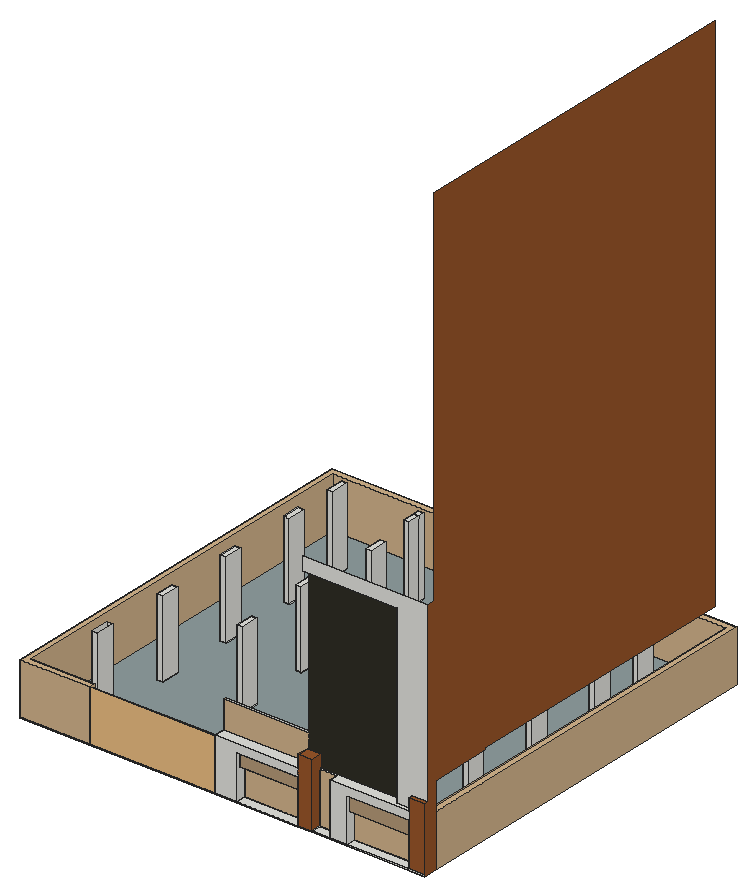
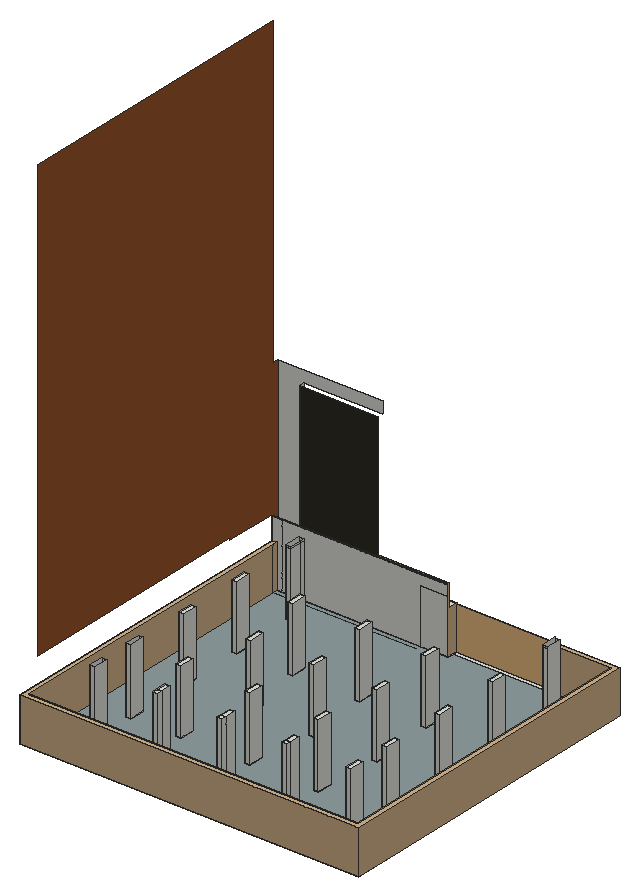
# SketchUp Ruby script. Lengths in inches.
U = 1.inch
M = Sketchup.active_model
def pt(a) = Geom::Point3d.new(a.map { |v| v * U })
def face(e, loops, mat)
  f = e.add_face(loops[0].map { |a| pt(a) })
  loops[1..].each { |l| e.add_face(l.map { |a| pt(a) }).erase! }
  f.material = f.back_material = mat if mat
  f
end
# faces: each face lists its corners as indices into pts; further lists are holes
def faces(e, pts, list, mat = nil) = list.each { |f| face(e, (f[0].is_a?(Array) ? f : [f]).map { |l| l.map { |i| pts[i] } }, mat) }
# xy, xz, yz: faces in a plane at the given z, y or x. An outline is a flat list of corners, or four numbers for a rectangle; further outlines are holes
def ring(l) = l.size == 4 ? [[l[0], l[1]], [l[2], l[1]], [l[2], l[3]], [l[0], l[3]]] : l.each_slice(2).to_a
def flat(e, list, mat, &to3) = list.each { |f| face(e, (f[0].is_a?(Array) ? f : [f]).map { |l| ring(l).map { |u, v| to3.(u, v) } }, mat) }
def xy(e, z, list, mat = nil) = flat(e, list, mat) { |x, y| [x, y, z] }
def xz(e, y, list, mat = nil) = flat(e, list, mat) { |x, z| [x, y, z] }
def yz(e, x, list, mat = nil) = flat(e, list, mat) { |y, z| [x, y, z] }
def lines(e, pts, list) = list.each { |a, b| e.add_line(pt(pts[a]), pt(pts[b])) }
# prism: a flat outline (further loops are holes) pulled along v
def prism(e, loops, v, mat = nil)
  f = face(e, loops, mat); d = Geom::Vector3d.new(v.map { |x| x * U })
  f.pushpull(f.normal.samedirection?(d) ? d.length : -d.length)
end
def box(e, o, s, mat = nil) = prism(e, [[o, [o[0] + s[0], o[1], o[2]], [o[0] + s[0], o[1] + s[1], o[2]], [o[0], o[1] + s[1], o[2]]]], [0, 0, s[2]], mat)
def at(x, y, z, deg = 0) = Geom::Transformation.translation(pt([x, y, z])) * Geom::Transformation.rotation(ORIGIN, Z_AXIS, deg.degrees)
def axes(o, x, y, z) = Geom::Transformation.new([*x, 0, *y, 0, *z, 0, *pt(o).to_a, 1])
def part(name) = M.definitions.add(name)
# library, detail: a bought-in or finely detailed component or shape, given as its bounding box
def library(name, o, s) = part(name).tap { |d| box(d.entities, o, s) }
def detail(e, o, s) = box(e.add_group.entities, o, s)
def put(e, d, t, mat = nil) = e.add_instance(d, t).tap { |i| i.material = mat if mat }
def group(e, t, mat = nil) = e.add_group.tap { |g| g.transformation = t; g.material = mat if mat }.entities
root = M.entities
M.materials.add("[0035_Tan]").color = [181, 154, 120]
M.materials.add("[0035_Tan]1").color = [210, 180, 140]
M.materials.add("[Metal Panel]").color = [143, 157, 158]
M.materials.add("[Stone Coursed Rough]").color = [48, 46, 38]
M.materials.add("[Wood Cherry Original]").color = [152, 86, 42]
c1 = library("gate (1)",[0,0,0],[171.26,1.97,78.74])
xy(root,0,[[0,2.9375,0,603.6875,623,603.6875,623,23.9375,299.4375,23.9375,299.4375,2.9375],[299.4375,2.9375,333.37,20.9375],[333.37,2.9375,428.37,17.9375],[428.37,2.9375,449.48,20.9375],[449.48,2.9375,476.56,17.9375],
  [476.56,2.9375,502.54,8.9375],[502.54,2.9375,598.64,17.9375],[598.64,2.9375,604.125,8.9375],[604.125,2.9375,623,8.9375],[476.56,8.9375,502.54,20.9375],
  [598.64,8.9375,604.125,20.9375],[604.125,8.9375,623,20.9375],[333.37,17.9375,428.37,17.9375,428.37,20.9375,449.48,20.9375,449.48,17.9375,476.56,17.9375,476.56,20.9375,502.54,20.9375,502.54,17.9375,598.64,17.9375,598.64,20.9375,604.125,20.9375,604.125,21.01,349.5625,23.9375,299.4375,23.9375,299.4375,20.9375,333.37,20.9375],[604.125,20.9375,610.875,20.9375,604.125,21.01],[610.875,20.9375,623,20.9375,623,23.9375,604.125,23.9375,604.125,21.01],
  [604.125,21.01,604.125,23.9375,349.5625,23.9375],[71.5,51.86,80.5,52.1875],[71.5,52.1875,80.5,80.1],[542.5,52.1875,551.5,80.43],[71.5,176.99,80.5,205.23],
  [194.375,176.99,203.375,205.23],[317.25,176.99,326.25,205.23],[440.125,176.99,449.125,205.23],[542.5,176.99,551.5,205.23],[71.5,298.8,80.5,327.04],
  [187.375,298.8,196.375,327.04],[303.25,298.8,312.25,327.04],[419.125,298.8,428.125,327.04],[542.5,298.8,551.5,327.04],[71.5,420.61,80.5,448.85],
  [198,420.61,207,448.85],[324.5,420.61,333.5,448.85],[451,420.61,460,448.85],[542.5,420.61,551.5,448.85],[71.5,503.93,80.5,532.16],
  [189.75,503.93,198.75,523.1875],[308,503.93,317,523.1875],[426.25,503.93,435.25,523.1875],[542.5,503.93,551.5,532.16],[189.75,523.1875,198.75,532.16],
  [308,523.1875,317,532.16],[426.25,523.1875,435.25,532.16]])
xy(root,0.4375,[[324.5,420.61,333.5,448.85]])
xy(root,1.625,[[108.02,2.9375,299.4375,11.9375],[333.37,2.9375,428.37,17.9375],[449.48,2.9375,476.56,17.9375],[502.54,2.9375,598.64,17.9375]])
xy(root,1.625,[[[9,11.9375,299.4375,11.9375,299.4375,23.9375,614,23.9375,614,594.6875,9,594.6875],[451,420.61,460,448.85],[324.5,420.61,333.5,448.85],[198,420.61,207,448.85],[71.5,503.93,80.5,532.16],[71.5,420.61,80.5,448.85],[189.75,503.93,198.75,532.16],[308,503.93,317,532.16],[426.25,503.93,435.25,532.16],[542.5,503.93,551.5,532.16],[542.5,420.61,551.5,448.85],[71.5,176.99,80.5,205.23],[419.125,298.8,428.125,327.04],[303.25,298.8,312.25,327.04],[187.375,298.8,196.375,327.04],[440.125,176.99,449.125,205.23],[317.25,176.99,326.25,205.23],[194.375,176.99,203.375,205.23],[71.5,51.86,80.5,80.1],[542.5,52.1875,551.5,80.43],[71.5,298.8,80.5,327.04],[542.5,298.8,551.5,327.04],[542.5,176.99,551.5,205.23]]],"[Metal Panel]")
xy(root,45.62,[[502.54,7.375,598.64,17.9375]],"[0035_Tan]")
xy(root,46.68,[[333.37,10.0625,428.37,17.9375]],"[0035_Tan]")
xy(root,69.21,[[333.37,2.9375,428.37,10.0625],[502.54,2.9375,598.64,7.375],[333.37,10.0625,428.37,20.9375]])
xy(root,80.37,[[0,2.9375,108.02,2.9375,108.02,11.9375,9,11.9375,9,594.6875,614,594.6875,614,23.9375,623,23.9375,623,603.6875,0,603.6875]],"[0035_Tan]1")
xy(root,81.17,[[299.4375,2.9375,428.37,20.9375],[476.56,2.9375,598.64,2.9375,598.64,9.86,574.78,9.86,574.78,20.9375,476.56,20.9375],[449.48,17.9375,476.56,20.9375]])
xy(root,100.11,[[428.37,2.9375,449.48,20.9375],[598.64,2.9375,623,9.86]],"[Wood Cherry Original]")
xy(root,120,[[71.5,176.99,80.5,205.23],[194.375,176.99,203.375,205.23],[317.25,176.99,326.25,205.23],[440.125,176.99,449.125,205.23],[542.5,176.99,551.5,205.23],
  [71.5,298.8,80.5,327.04],[187.375,298.8,196.375,327.04],[303.25,298.8,312.25,327.04],[419.125,298.8,428.125,327.04],[542.5,298.8,551.5,327.04],
  [71.5,420.61,80.5,448.85],[198,420.61,207,448.85],[324.5,420.61,333.5,448.85],[451,420.61,460,448.85],[71.5,503.93,80.5,532.16],
  [189.75,503.93,198.75,523.1875],[189.75,503.93,198.75,523.1875],[189.75,503.93,198.75,523.1875],[308,503.93,317,523.1875],[308,503.93,317,523.1875],
  [308,503.93,317,523.1875],[426.25,503.93,435.25,523.1875],[426.25,503.93,435.25,523.1875],[426.25,503.93,435.25,523.1875],[189.75,523.1875,198.75,532.16],
  [308,523.1875,317,532.16],[426.25,523.1875,435.25,532.16]])
xz(root,2.9375,[[0,0,299.4375,1.625],[299.4375,0,333.37,1.625],[333.37,0,428.37,1.625],[449.48,0,476.56,1.625],[476.56,0,623,1.625],
  [299.4375,1.625,333.37,1.625,333.37,69.21,428.37,69.21,428.37,81.17,299.4375,81.17],[476.56,1.625,502.54,1.625,502.54,69.21,598.64,69.21,598.64,81.17,476.56,81.17]])
xz(root,2.9375,[[0,1.625,108.02,80.37]],"[0035_Tan]1")
xz(root,2.9375,[[428.37,1.625,449.48,100.11],[598.64,1.625,623,100.11]],"[Wood Cherry Original]")
xz(root,7.375,[[502.54,45.62,598.64,69.21]],"[0035_Tan]")
xz(root,9.86,[[574.78,81.17,598.64,81.17,598.64,100.11,623,100.11,623,372,430.625,372,430.625,350.47,574.78,350.47]])
xz(root,10.0625,[[333.37,46.68,428.37,69.21]],"[0035_Tan]")
xz(root,11.9375,[[9,1.625,108.02,80.37]],"[0035_Tan]1")
xz(root,17.9375,[[333.37,0,428.37,1.625],[449.48,0,476.56,1.625],[502.54,0,598.64,1.625]])
xz(root,17.9375,[[333.37,1.625,428.37,46.68],[449.48,1.625,476.56,81.17],[502.54,1.625,598.64,45.62]],"[0035_Tan]1")
xz(root,20.9375,[[299.4375,81.17,428.37,81.17,428.37,100.11,430.625,100.11,430.625,123,299.4375,123]],"[0035_Tan]1")
xz(root,20.9375,[[449.48,81.17,574.78,81.17,574.78,350.47,430.625,350.47,430.625,100.11,449.48,100.11]],"[Stone Coursed Rough]")
xz(root,23.9375,[[299.4375,0,349.5625,1.625],[349.5625,0,604.125,1.625],[604.125,0,623,1.625],[299.4375,1.625,349.5625,101.29],[349.5625,1.625,349.5625,101.29,299.4375,101.29,299.4375,120,604.125,120,604.125,1.625],
  [604.125,1.625,604.125,120,623,120,623,80.37,614,80.37,614,1.625],[614,1.625,623,80.37],[299.4375,120,604.125,123],[604.125,120,623,123]])
xz(root,51.86,[[71.5,0,80.5,1.625]])
xz(root,52.1875,[[71.5,0,80.5,123],[542.5,0,551.5,1.625],[542.5,1.625,551.5,123]])
xz(root,80.1,[[71.5,0,80.5,1.625],[71.5,1.625,80.5,120],[71.5,120,80.5,123.75]])
xz(root,80.43,[[542.5,0,551.5,1.625],[542.5,1.625,551.5,120],[542.5,120,551.5,123]])
xz(root,176.99,[[71.5,0,80.5,1.625],[194.375,0,203.375,1.625],[317.25,0,326.25,1.625],[440.125,0,449.125,1.625],[542.5,0,551.5,1.625],
  [71.5,1.625,80.5,120],[194.375,1.625,203.375,120],[317.25,1.625,326.25,120],[440.125,1.625,449.125,120],[542.5,1.625,551.5,120]])
xz(root,205.23,[[71.5,0,80.5,1.625],[194.375,0,203.375,1.625],[317.25,0,326.25,1.625],[440.125,0,449.125,1.625],[542.5,0,551.5,1.625],
  [71.5,1.625,80.5,120],[194.375,1.625,203.375,120],[317.25,1.625,326.25,120],[440.125,1.625,449.125,120],[542.5,1.625,551.5,120]])
xz(root,298.8,[[71.5,0,80.5,1.625],[187.375,0,196.375,1.625],[303.25,0,312.25,1.625],[419.125,0,428.125,1.625],[542.5,0,551.5,1.625],
  [71.5,1.625,80.5,120],[187.375,1.625,196.375,120],[303.25,1.625,312.25,120],[419.125,1.625,428.125,120],[542.5,1.625,551.5,120]])
xz(root,327.04,[[71.5,0,80.5,1.625],[187.375,0,196.375,1.625],[303.25,0,312.25,1.625],[419.125,0,428.125,1.625],[542.5,0,551.5,1.625],
  [71.5,1.625,80.5,120],[187.375,1.625,196.375,120],[303.25,1.625,312.25,120],[419.125,1.625,428.125,120],[542.5,1.625,551.5,120]])
xz(root,420.61,[[71.5,0,80.5,1.625],[198,0,207,1.625],[324.5,0,333.5,0.4375],[451,0,460,1.625],[542.5,0,551.5,1.625],
  [324.5,0.4375,333.5,1.625],[71.5,1.625,80.5,120],[198,1.625,207,120],[324.5,1.625,333.5,120],[451,1.625,460,120],
  [542.5,1.625,551.5,123]])
xz(root,448.85,[[71.5,0,80.5,1.625],[198,0,207,1.625],[324.5,0,333.5,0.4375],[451,0,460,1.625],[542.5,0,551.5,1.625],
  [324.5,0.4375,333.5,1.625],[71.5,1.625,80.5,120],[198,1.625,207,120],[324.5,1.625,333.5,120],[451,1.625,460,120],
  [542.5,1.625,551.5,123]])
xz(root,503.93,[[71.5,0,80.5,1.625],[189.75,0,198.75,1.625],[308,0,317,1.625],[426.25,0,435.25,1.625],[542.5,0,551.5,1.625],
  [71.5,1.625,80.5,120],[189.75,1.625,198.75,120],[308,1.625,317,120],[426.25,1.625,435.25,120],[542.5,1.625,551.5,123]])
xz(root,523.1875,[[189.75,0,198.75,120],[308,0,317,120],[426.25,0,435.25,120]])
xz(root,532.16,[[71.5,0,80.5,1.625],[189.75,0,198.75,1.625],[308,0,317,1.625],[426.25,0,435.25,1.625],[542.5,0,551.5,1.625],
  [71.5,1.625,80.5,120],[189.75,1.625,198.75,120],[308,1.625,317,120],[426.25,1.625,435.25,120],[542.5,1.625,551.5,123]])
xz(root,594.6875,[[9,1.625,614,80.37]],"[0035_Tan]1")
xz(root,603.6875,[[0,0,623,80.37]],"[0035_Tan]1")
yz(root,0,[[2.9375,0,603.6875,80.37]],"[0035_Tan]1")
yz(root,9,[[11.9375,1.625,594.6875,80.37]],"[0035_Tan]1")
yz(root,71.5,[[51.86,0,52.1875,1.625],[52.1875,0,80.1,1.625],[176.99,0,205.23,1.625],[298.8,0,327.04,1.625],[420.61,0,448.85,1.625],
  [503.93,0,532.16,1.625],[532.16,0,532.1875,1.625],[52.1875,1.625,80.1,123],[176.99,1.625,205.23,120],[298.8,1.625,327.04,120],
  [420.61,1.625,448.85,120],[503.93,1.625,532.16,120]])
yz(root,80.5,[[51.86,0,52.1875,1.625],[52.1875,0,80.1,1.625],[176.99,0,205.23,1.625],[298.8,0,327.04,1.625],[420.61,0,448.85,1.625],
  [503.93,0,523.1875,1.625],[523.1875,0,532.16,1.625],[52.1875,1.625,80.1,123.75],[176.99,1.625,205.23,120],[298.8,1.625,327.04,120],
  [420.61,1.625,448.85,120],[503.93,1.625,532.16,120]])
yz(root,108.02,[[2.9375,1.625,11.9375,80.37]],"[0035_Tan]1")
yz(root,187.375,[[298.8,0,327.04,1.625],[298.8,1.625,327.04,120]])
yz(root,189.75,[[503.93,0,523.1875,1.625],[523.1875,0,532.16,1.625],[503.93,1.625,523.1875,120],[523.1875,1.625,532.16,120]])
yz(root,194.375,[[176.99,0,205.23,1.625],[176.99,1.625,205.23,120]])
yz(root,196.375,[[298.8,0,327.04,1.625],[298.8,1.625,327.04,120]])
yz(root,198,[[420.61,0,448.85,1.625],[420.61,1.625,448.85,120]])
yz(root,198.75,[[503.93,0,523.1875,1.625],[523.1875,0,532.16,1.625],[503.93,1.625,523.1875,120],[523.1875,1.625,532.16,120]])
yz(root,203.375,[[176.99,0,205.23,1.625],[176.99,1.625,205.23,120]])
yz(root,207,[[420.61,0,448.85,1.625],[420.61,1.625,448.85,120]])
yz(root,299.4375,[[2.9375,0,20.9375,1.625],[20.9375,0,23.9375,1.625]])
yz(root,299.4375,[[2.9375,1.625,2.9375,81.17,20.9375,81.17,20.9375,123,23.9375,123,23.9375,1.625]],"[0035_Tan]1")
yz(root,303.25,[[298.8,0,327.04,1.625],[298.8,1.625,327.04,120]])
yz(root,308,[[503.93,0,523.1875,1.625],[523.1875,0,532.16,1.625],[503.93,1.625,523.1875,120],[523.1875,1.625,532.16,120]])
yz(root,312.25,[[298.8,0,327.04,1.625],[298.8,1.625,327.04,120]])
yz(root,317,[[503.93,0,523.1875,1.625],[523.1875,0,532.16,1.625],[503.93,1.625,523.1875,120],[523.1875,1.625,532.16,120]])
yz(root,317.25,[[176.99,0,205.23,1.625],[176.99,1.625,205.23,120]])
yz(root,324.5,[[420.61,0,448.85,0.4375],[420.61,0.4375,448.85,1.625],[420.61,1.625,448.85,120]])
yz(root,326.25,[[176.99,0,205.23,1.625],[176.99,1.625,205.23,120]])
yz(root,333.37,[[2.9375,0,17.9375,1.625],[17.9375,0,20.9375,0,20.9375,69.21,10.0625,69.21,10.0625,46.68,17.9375,46.68],[2.9375,1.625,17.9375,1.625,17.9375,46.68,10.0625,46.68,10.0625,69.21,2.9375,69.21]])
yz(root,333.5,[[420.61,0,448.85,0.4375],[420.61,0.4375,448.85,1.625],[420.61,1.625,448.85,120]])
yz(root,419.125,[[298.8,0,327.04,1.625],[298.8,1.625,327.04,120]])
yz(root,426.25,[[503.93,0,523.1875,1.625],[523.1875,0,532.16,1.625],[503.93,1.625,523.1875,120],[523.1875,1.625,532.16,120]])
yz(root,428.125,[[298.8,0,327.04,1.625],[298.8,1.625,327.04,120]])
yz(root,428.37,[[2.9375,0,17.9375,1.625],[17.9375,0,17.9375,46.68,10.0625,46.68,10.0625,69.21,20.9375,69.21,20.9375,0]])
yz(root,428.37,[[2.9375,1.625,2.9375,69.21,10.0625,69.21,10.0625,46.68,17.9375,46.68,17.9375,1.625],[2.9375,81.17,20.9375,100.11]],"[Wood Cherry Original]")
yz(root,435.25,[[503.93,0,523.1875,1.625],[523.1875,0,532.16,1.625],[503.93,1.625,523.1875,120],[523.1875,1.625,532.16,120]])
yz(root,440.125,[[176.99,0,205.23,1.625],[176.99,1.625,205.23,120]])
yz(root,449.125,[[176.99,0,205.23,1.625],[176.99,1.625,205.23,120]])
yz(root,449.48,[[2.9375,0,17.9375,1.625],[17.9375,0,20.9375,81.17]])
yz(root,449.48,[[2.9375,1.625,17.9375,1.625,17.9375,81.17,20.9375,81.17,20.9375,100.11,2.9375,100.11]],"[Wood Cherry Original]")
yz(root,451,[[420.61,0,448.85,1.625],[420.61,1.625,448.85,120]])
yz(root,460,[[420.61,0,448.85,1.625],[420.61,1.625,448.85,120]])
yz(root,476.56,[[2.9375,0,8.9375,1.625],[8.9375,0,17.9375,1.625],[2.9375,1.625,17.9375,81.17]])
yz(root,502.54,[[8.9375,0,17.9375,1.625],[2.9375,1.625,17.9375,1.625,17.9375,45.62,7.375,45.62,7.375,69.21,2.9375,69.21]])
yz(root,542.5,[[52.1875,0,61.1875,1.625],[61.1875,0,80.43,1.625],[176.99,0,205.23,1.625],[298.8,0,327.04,1.625],[420.61,0,448.85,1.625],
  [503.93,0,523.1875,1.625],[523.1875,0,532.16,1.625],[52.1875,1.625,61.1875,120],[61.1875,1.625,80.43,120],[176.99,1.625,205.23,120],
  [298.8,1.625,327.04,120],[420.61,1.625,448.85,123],[503.93,1.625,532.16,123],[52.1875,120,61.1875,123],[61.1875,120,80.43,123]])
yz(root,551.5,[[52.1875,0,80.43,1.625],[176.99,0,205.23,1.625],[298.8,0,327.04,1.625],[420.61,0,448.85,1.625],[503.93,0,532.16,1.625],
  [532.16,0,532.1875,1.625],[52.1875,1.625,80.43,123],[176.99,1.625,205.23,120],[298.8,1.625,327.04,120],[420.61,1.625,448.85,123],
  [503.93,1.625,532.16,123]])
yz(root,574.78,[[9.86,81.17,20.9375,350.47]])
yz(root,598.64,[[8.9375,0,17.9375,1.625]])
yz(root,598.64,[[2.9375,1.625,2.9375,69.21,7.375,69.21,7.375,45.62,17.9375,45.62,17.9375,1.625],[2.9375,81.17,9.86,100.11]],"[Wood Cherry Original]")
yz(root,614,[[23.9375,1.625,32.9375,80.37],[32.9375,1.625,594.6875,80.37]],"[0035_Tan]1")
yz(root,623,[[23.9375,0,603.6875,80.37]],"[0035_Tan]1")
yz(root,623,[[2.9375,0,23.9375,0,23.9375,123,119.9375,123,119.9375,126,561.98,126,561.98,936,20.9375,936,20.9375,372,9.86,372,9.86,100.11,2.9375,100.11]],"[Wood Cherry Original]")
p = [[71.5,205.23,0],[71.5,298.8,0],[71.5,80.1,0],[71.5,176.99,0],[71.5,327.04,0],[71.5,420.61,0],
  [551.5,176.99,0],[551.5,80.43,0],[551.5,298.8,0],[551.5,205.23,0],[551.5,503.93,0],[551.5,448.85,0],
  [542.5,52.1875,0],[80.5,52.1875,0],[604.125,23.9375,120],[604.125,20.9375,120],[574.78,20.9375,81.17],[610.875,20.9375,81.17],
  [598.64,9.86,81.17],[610.875,9.86,81.17],[349.5625,32.9375,0],[604.125,32.9375,0],[614,32.9375,0],[614,594.6875,0],
  [9,594.6875,0],[551.5,327.04,0],[551.5,420.61,0],[71.5,503.93,0],[71.5,448.85,0],[349.5625,32.9375,1.625],
  [604.125,32.9375,1.625],[614,32.9375,1.625]]
lines(root,p,[[0,1],[2,3],[4,5],[6,7],[8,9],[10,11],[12,13],[14,15],[16,17],[18,19],[20,21],[21,22],
  [22,23],[23,24],[25,26],[27,28],[29,30],[30,31]])
put(root,c1,axes([108.02,2.9375,1.625],[1.12,0,0],[0,1,0],[0,0,1]))
